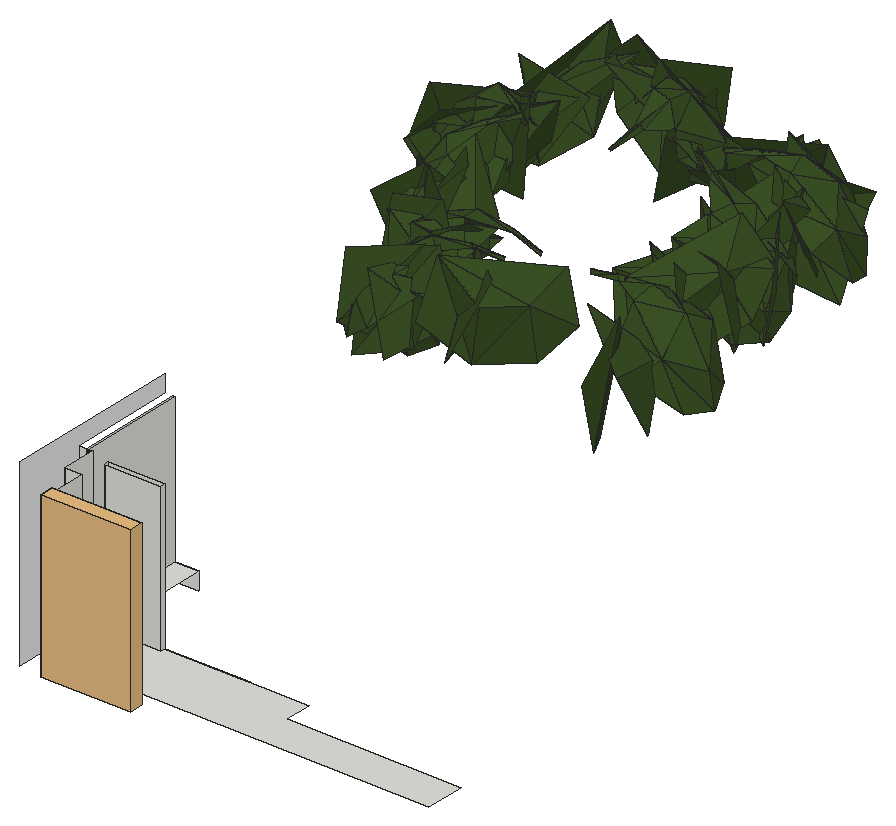
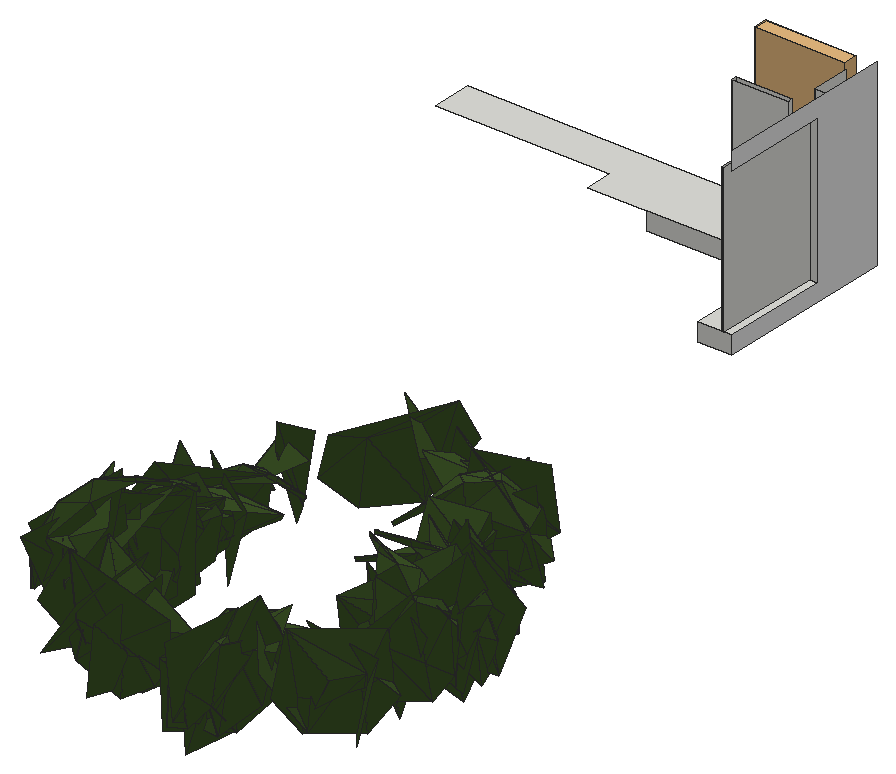
# SketchUp Ruby script. Lengths in inches.
U = 1.inch
M = Sketchup.active_model
def pt(a) = Geom::Point3d.new(a.map { |v| v * U })
def face(e, loops, mat)
  f = e.add_face(loops[0].map { |a| pt(a) })
  loops[1..].each { |l| e.add_face(l.map { |a| pt(a) }).erase! }
  f.material = f.back_material = mat if mat
  f
end
# faces: each face lists its corners as indices into pts; further lists are holes
def faces(e, pts, list, mat = nil) = list.each { |f| face(e, (f[0].is_a?(Array) ? f : [f]).map { |l| l.map { |i| pts[i] } }, mat) }
# xy, xz, yz: faces in a plane at the given z, y or x. An outline is a flat list of corners, or four numbers for a rectangle; further outlines are holes
def ring(l) = l.size == 4 ? [[l[0], l[1]], [l[2], l[1]], [l[2], l[3]], [l[0], l[3]]] : l.each_slice(2).to_a
def flat(e, list, mat, &to3) = list.each { |f| face(e, (f[0].is_a?(Array) ? f : [f]).map { |l| ring(l).map { |u, v| to3.(u, v) } }, mat) }
def xy(e, z, list, mat = nil) = flat(e, list, mat) { |x, y| [x, y, z] }
def xz(e, y, list, mat = nil) = flat(e, list, mat) { |x, z| [x, y, z] }
def yz(e, x, list, mat = nil) = flat(e, list, mat) { |y, z| [x, y, z] }
def lines(e, pts, list) = list.each { |a, b| e.add_line(pt(pts[a]), pt(pts[b])) }
# prism: a flat outline (further loops are holes) pulled along v
def prism(e, loops, v, mat = nil)
  f = face(e, loops, mat); d = Geom::Vector3d.new(v.map { |x| x * U })
  f.pushpull(f.normal.samedirection?(d) ? d.length : -d.length)
end
def box(e, o, s, mat = nil) = prism(e, [[o, [o[0] + s[0], o[1], o[2]], [o[0] + s[0], o[1] + s[1], o[2]], [o[0], o[1] + s[1], o[2]]]], [0, 0, s[2]], mat)
def at(x, y, z, deg = 0) = Geom::Transformation.translation(pt([x, y, z])) * Geom::Transformation.rotation(ORIGIN, Z_AXIS, deg.degrees)
def axes(o, x, y, z) = Geom::Transformation.new([*x, 0, *y, 0, *z, 0, *pt(o).to_a, 1])
def part(name) = M.definitions.add(name)
# library, detail: a bought-in or finely detailed component or shape, given as its bounding box
def library(name, o, s) = part(name).tap { |d| box(d.entities, o, s) }
def detail(e, o, s) = box(e.add_group.entities, o, s)
def put(e, d, t, mat = nil) = e.add_instance(d, t).tap { |i| i.material = mat if mat }
def group(e, t, mat = nil) = e.add_group.tap { |g| g.transformation = t; g.material = mat if mat }.entities
root = M.entities
M.materials.add("AM113_062_Tilia").color = [58, 81, 37]
M.materials.add("white_wall").color = [233, 233, 233]
c1 = library("Shrub+_Grass",[-121.83,-22.34,0],[123.96,19.94,123.95])
xy(root,297.35,[[413.32,28.625,935.92,28.625,935.92,83.29,695.48,83.29,695.48,121.6875,496.21,121.6875,496.21,115.3125,418.81,115.3125,418.81,278.26,385.62,278.26,385.62,130.3125,390.32,130.3125,390.32,82.67,413.32,82.67],[418.81,115.3125,496.21,121.6875],[371.87,130.3125,382.06,278.26],[382.06,130.3125,385.62,278.26]])
xz(root,82.67,[[390.32,297.35,413.32,500.91]])
xz(root,115.3125,[[418.81,297.35,496.21,500.91]])
xz(root,121.6875,[[496.21,273.04,613.65,297.35],[418.81,297.35,496.21,500.91]])
xz(root,130.3125,[[371.87,297.35,382.06,500.91],[382.06,297.35,385.62,500.91],[385.62,297.35,390.32,500.91]])
xz(root,278.26,[[371.87,273.04,418.81,297.35],[382.06,297.35,385.62,500.91]])
yz(root,371.87,[[28.625,273.04,28.625,525.1,278.26,525.1,278.26,500.91,130.3125,500.91,130.3125,297.35,278.26,297.35,278.26,273.04]],"white_wall")
yz(root,382.06,[[130.3125,297.35,278.26,500.91]])
yz(root,385.62,[[130.3125,297.35,278.26,500.91]])
yz(root,390.32,[[82.67,297.35,130.3125,500.91]])
yz(root,413.32,[[28.625,297.35,82.67,500.91]])
yz(root,418.81,[[115.3125,297.35,121.6875,500.91]])
yz(root,496.21,[[115.3125,297.35,121.6875,500.91]])
p = [[565.42,1074.05,347.14],[473.11,1076.04,429.39],[517.03,1076.78,251.14],[451.75,1104.5,310.63],[124.09,980.42,346.32],[174.26,1054.83,429.43],
  [142.82,1026.51,253.56],[201.08,1066.89,309.96],[542.4,803.89,256.72],[526.35,835.0625,255.56],[521.17,877.52,364.75],[204.78,925.17,256.16],
  [226.65,870.02,314.07],[218.93,918.58,365.5],[200.1875,963.85,327.84],[236.73,1028.86,315.61],[184.69,1005.02,258.76],[529.41,865.28,392.49],
  [539.14,787.86,344.57],[560.75,821.36,346.28],[565.625,868.44,257.36],[543.39,920.94,325.3],[557.08,902.7,333.4375],[580.49,912.46,269.3],
  [588.52,955.39,257.48],[585.34,950.82,307.52],[576.85,986.33,274.56],[268.35,895.48,383.67],[270.83,858.14,265.86],[220.66,790.14,270.84],
  [182.18,990.33,313.11],[157.6,954.42,268.03],[158.1,911.76,284.91],[196.71,1003.23,274.22],[140.53,985.93,269.15],[162.25,965.33,292.7],
  [127.97,985.77,316.2],[115.83,1037.13,348.44],[119.67,1023.7,279.89],[535.94,880.77,309],[440.12,1029.02,382.82],[481.72,1009.85,270.04],
  [536.36,947.3,290.85],[518.68,1039.48,342.86],[530.18,1055.24,275.41],[554.09,1092.74,270.55],[559.36,1077.5625,316.66],[561.57,1119.85,298.74],
  [232.85,789.04,384.3125],[140.57,950.14,352.37],[190.2,974.27,273.55],[236.15,982.17,351.65],[310.18,1219.3,383.75],[269.26,1249.37,274.58],
  [281.45,1333.08,273.91],[291.21,1329.84,387.71],[246.46,993.13,313.43],[555.97,993,341.74],[518.39,1024.73,340.52],[289.46,790.39,377.59],
  [237.56,799.57,345.67],[272.73,819.99,274.86],[332.7,798.7,318.77],[196.34,847.78,367.41],[191.52,826.9,289],[546.44,1120.36,421.7],
  [586.46,1062.82,356.48],[559.14,1076.29,275.13],[526.65,1124.94,400.61],[528.91,1091.98,285.93],[485.8,1034.11,325.7],[177.74,971.25,413.4],
  [105.18,966.85,356.36],[124.28,988.9,275.76],[189.57,987.47,392.76],[152.64,1007.23,285.1],[418.84,1319.11,379.39],[439.56,1305.13,276.45],
  [389.36,1247.37,293.16],[470.83,1253.625,285.62],[399.27,1259.62,276.43],[408.0625,1287.39,349.05],[354.28,1271.51,311.54],[480.33,1272.95,294.44],
  [408.32,1286.3,277.53],[409.71,1275.94,358.07],[361.54,1288.3,309.81],[516.07,1024.48,357.375],[499.64,1036.16,278.41],[486.36,1116.42,293.93],
  [147.64,925.03,291.07],[181.33,926.36,278.61],[241.63,929.63,372.95],[346.58,1295.18,353.86],[326.71,1314.76,278.91],[251.58,1282.1875,288.58],
  [255.6,805.6,278.97],[316.54,775.61,318.15],[288.3,803.46,381.79],[239.32,826.95,359.37],[222.83,900.29,359.07],[190.1875,851.45,304.82],
  [175.07,1024.77,279.71],[215.3,966.87,305.31],[177.61,975.15,368.4375],[142.8,1017.9,354.66],[140.06,1082.25,401.69],[116.41,1073.2,315.95],
  [125.43,1069.0625,333.45],[465.625,1034.93,394.92],[486.8,1025.62,306.64],[502.52,1104.04,281.29],[522.74,1072.12,354.01],[543.91,1122.28,375.93],
  [534.38,1165.23,317.22],[584.42,1102.64,358.01],[540.49,1142.12,281.66],[509.74,1172.49,364.83],[470.93,947.34,384.19],[493.29,929.2,309.82],
  [518.91,1004.47,282.71],[528,974.23,360.85],[547.36,1025.99,384.49],[551.39,1062.78,318.11],[176.99,893.1875,315.62],[163.21,934.92,325.15],
  [465.66,1291.55,358.61],[499.27,1261.56,420.2],[532.42,1274.12,350.76],[105.04,1045.5,364.82],[117.67,1058.8,286.46],[194.12,1032.34,290.86],
  [173.24,914.7,379.5],[197.41,877.89,287.8],[265.34,886.15,335.07],[198.48,1273.14,350.54],[242.27,1301.75,396.73],[285.03,1317.81,350.16],
  [204.99,1115.18,442.68],[201.84,1106.86,317.86],[133.52,1149.07,289.38],[103.75,1139,394.64],[346.81,1236.28,346.6],[342.13,1293.99,290.875],
  [260.27,1303.03,289.6],[298.73,1293.05,360.57],[201.45,1301.11,348.3125],[250.09,1290.84,398.875],[535.63,971.84,400.95],[177.58,965.8,356.21],
  [140.22,1001.44,324.09],[233.68,980.02,326.08],[232.74,931.4,404.49],[150.63,947.48,376.5625],[426.15,983.3,365.78],[468.47,935.03,323.04],
  [528.875,985.3,291.24],[501.21,983.41,371.14],[534.21,1028.18,387.43],[570.23,1042.13,322.73],[210.93,958.6,382.64],[164.91,963.76,364.36],
  [419.77,1201.3125,388.88],[442.71,1195.97,406.0625],[483.45,1217.41,293.45],[509.33,1297.54,303.9375],[539.3,1080.3125,324.46],[552.52,1127.77,364.5],
  [513.36,1173.52,338.95],[463.64,1266.77,378.92],[491.1875,1203.03,416.06],[531.48,1253.21,373.72],[523.09,1139.91,457.67],[519.49,1132.15,330.84],
  [591.36,1168.09,296.72],[595.41,1211.44,396.58],[148.9,1201.36,298.59],[130.5,1157.85,332.11],[127.95,1211.69,374.61],[169.52,1269.79,311.48],
  [259.3,769.38,400.81],[285.56,763.64,298.66],[338.32,812.03,337.35],[560.28,1116.76,371.51],[542.35,1158.59,395.58],[329.71,1300.86,345.54],
  [336.4,1283.18,306.22],[304.24,1336.92,301.48],[264.22,1351.13,319.19],[124.7,1215.33,303.35],[115.4375,1168.3,332.79],[140.02,1210.64,382.35],
  [153.0625,1282.39,323.1],[580.81,1243.58,398.83],[545.72,1225.25,303.81],[484.52,1220.6,365.09],[451.14,1307.125,389.6],[219.18,765.42,320.9],
  [241.2,789.54,304.42],[299.26,826.3,388.73],[206.67,835.57,354.34],[203.98,795.28,304.625],[234.38,762.87,310.03],[202.77,857.17,317.74],
  [222.12,933.99,356.98],[148.71,1116.59,306.13],[116.23,1054.54,333.8],[122.6,1086.16,402.59],[145.76,1136.13,388.46],[211.85,1159.8125,418.71],
  [178.29,1185.79,345.08],[309.91,1239.64,345],[100.96,1226.86,409.14],[112.4375,1249.61,306.4],[159.93,1188.44,313.2],[547.72,956.81,363.52],
  [83.67,1111.39,403.31],[107.58,1083.3,308.36],[146.61,1037.31,368.88],[335.17,861.17,413.37],[346.14,806.08,308.68],[389.2,738.24,342.82],
  [494.05,913.92,341.8125],[164.55,1101.23,309.81],[138.74,1041.11,345.54],[111.78,1083.61,393.14],[124.02,1134.8,363.83],[158.99,1180.49,401.77],
  [159.98,1181.6875,319.94],[353.26,1227.36,351.68],[265.27,759.75,332.54],[230.01,781.04,354.46],[560.0625,995,414.84],[575.67,1007.41,310.08],
  [538.94,1073.21,334.06],[382.68,793.49,313.49],[432.64,845.53,311.05],[435.63,828.28,389.64],[463.07,876.98,351.67],[135.91,1268.4,388.18],
  [358.56,1263.54,380.97],[175.64,1292.39,448.04],[165.7,1330.77,382.49],[559.6,1109.25,440.05],[600.6,1117.37,364.04],[554.76,1172.62,311.98],
  [572.07,1175.27,396.56],[515.52,1234.72,327.23],[539.12,1221.7,401.12],[280.37,1356.24,325.22],[269.76,1324.34,312.32],[252.59,1265.63,405.83],
  [204.46,956.31,369.4],[247.74,991.84,351.14],[216.8,1204.48,404.96],[347.79,778.22,444.4375],[349.14,738.3125,379.18],[401.84,781.17,396.57],
  [237.98,860.38,379.8125],[99.35,1133.52,314.8],[93.3,1103.35,336.5],[103.99,1140.44,363.4],[152.11,1168.9,385.16],[127.88,1166.51,321.61],
  [597.96,1153.28,398.18],[609.04,1168.27,330.3125],[594.16,1208.65,315.06],[597.12,1206.875,365.41],[570.08,1231.25,332.27],[202.74,915.69,373.65],
  [245.96,893.42,383.27],[286.1,906.75,404.6],[145.5,995.08,384.94],[541.24,1082.78,387.08],[559.46,1182.5,373.32],[252.48,880.33,346.4],
  [341.91,771.98,378.12],[564.95,1086.46,378.09],[352.45,786.75,381.62],[284.49,1337.82,358.91],[240.5,1339.56,350.03],[296.76,819.8,421.14],
  [221.16,778.91,409.52],[181.27,1174.29,360.42],[577.08,1072.7,378.02],[160.95,1260.6,405.38],[230.96,1273.36,436.63],[187.35,1324.65,402.84],
  [257.62,1273,437.4375],[301.08,1344.65,410.22],[466.5,888.41,376.58],[471.67,1070.36,383.2],[233.24,941.21,372.79],[501.54,1267.84,377.62],
  [588.67,1122.17,378.51],[143.38,1157.01,400.51],[553.38,1232.02,401.89],[505.17,1241.48,405.11],[279.51,790.07,391.25],[327.29,801.63,388.86],
  [175.88,1146.29,366.84],[497.9,928.74,374.03],[167.03,1061.3,385.09],[99.37,1030.38,389.49],[458.14,1049.2,383.12],[273.53,975.64,363.21],
  [122.52,1047.93,411.18],[107.01,1093.55,404.89],[291.87,882.28,386.62],[547.34,1187.59,389.81],[493.73,986.29,341.62],[507.53,977.93,373.27],
  [417.13,785.98,432.45],[488.14,1073.95,414.11],[325.2,984.35,344.57],[283.95,985.58,358.36],[288.24,983.82,365.24],[326.75,985.04,349.57],
  [308.58,1238.47,382.72],[112.97,1021.65,399.88],[290.53,1291.21,402.21],[260.47,877.93,382.625],[291.24,978.7,363.01],[325.64,981.89,346.5],
  [215.91,1231.58,437.36],[189.03,1293.11,414.09],[164.44,1043.63,414.3],[217.24,1274.08,416.8],[253.1,1306.93,407.28],[187.52,1275.17,418.59],
  [245.63,975.03,378.875],[442.29,884.58,416.02],[192.7,1035.61,428.46],[231.34,1267.91,459.49],[254.15,821.66,397.31],[261.98,930.65,356.1],
  [248.65,947.68,381.73],[198.66,949.72,424.68],[234.41,972.27,428.45],[555.38,1148.27,437.51],[481.42,1101.7,432.33],[351.98,836.91,407.47],
  [199.45,1128.51,400.53],[132.23,1121.73,422.3125],[321.45,924.22,363.5],[292.43,896.89,382.99],[297.86,898.01,388.64],[322.98,925.46,368.32],
  [506.06,952.68,387.53],[207.64,1002.96,391.28],[184.85,998.7,413.5625],[302.99,896.34,384.74],[323.67,922.57,364.68],[506.97,1161.17,451.78],
  [565.46,1198.15,426.71],[515.01,1099.81,398.31],[325.29,810.4375,434.49],[194.16,1090.85,441.4],[310.88,841.6,369.74],[294.375,843.85,400.94],
  [422.66,949.15,371.29],[464.48,944.32,380],[461.45,949.2,385.33],[421.69,950.66,376.23],[458.99,953.45,380.49],[422.84,952.05,371.48],
  [518.48,1113.59,420],[504.13,1133.78,399.64],[517.92,1169.01,443.11],[287.0625,1203.15,396.46],[274.65,1166.81,380.29],[274.5,1168.56,375.32],
  [290.15,1206.64,389.6],[281.2,1202.15,394.3],[272.05,1168.98,377.29],[471.86,1229.28,441.6875],[533.66,1071.42,432.41],[538.39,1133.32,416.1],
  [274.21,862.35,405.61],[293.79,1246,410.8],[168.35,1018.33,425.16],[188.42,1121.08,433.54],[508.65,1088.55,427.96],[246.32,1246.4,388.7],
  [267.14,1252.67,414.16],[152.27,1027.71,445.43],[118.4375,1051.59,457],[536.71,1150.49,446.64],[502.68,1196.2,412.1875],[520.94,1197.92,441.77],
  [162.87,1067.77,409.6],[155.26,1084.7,438.2],[205.64,1044.02,439.63],[467.88,1098.36,439.08],[196.58,1048.49,435.96],[467.4375,1108.24,444.23],
  [169.26,1106.42,449.04],[200.24,1045.59,442.625],[533.01,1176.29,457.45],[468.58,1102.42,446.49],[208.61,1091.75,444.42],[232.63,1068.24,446.92],
  [208.57,1081.38,446.56],[432.64,1120.08,452.24],[232.97,1066.99,452.02],[234.07,1065.77,447.26],[208.63,1086.64,450.52],[241.46,1064.52,445.45],
  [241.45,1065.8,440.34],[239.8125,1063.48,440.875],[491.32,1153.76,458.05],[433.5,1120.53,457.55],[434.15,1122.5,452.98],[500.52,1148.41,457.15],
  [495.88,1151.6,462.67],[460.05,1133.04,460.01],[461.28,1131.82,455.03],[460.03,1134.46,455.04]]
faces(root,p,[[0,1,2],[1,3,2],[4,5,6],[5,7,6],[8,9,10],[11,12,13],[13,14,11],[15,16,11],
  [11,14,15],[17,18,8],[10,17,8],[19,20,21],[22,23,24],[24,25,22],[24,26,25],[27,28,29],
  [30,31,32],[30,33,31],[34,35,36],[34,36,37],[37,38,34],[22,39,23],[40,41,42],[43,44,45],
  [45,46,43],[45,47,46],[48,27,29],[49,50,51],[52,53,54],[55,52,54],[56,33,30],[25,26,57],
  [26,58,57],[59,60,61],[61,62,59],[61,60,63],[63,64,61],[65,66,67],[68,65,67],[67,69,68],
  [43,70,44],[71,72,73],[74,71,73],[73,75,74],[76,77,78],[79,80,81],[80,82,81],[83,84,85],
  [84,86,85],[87,88,89],[90,91,92],[93,94,95],[96,97,98],[98,99,96],[100,101,96],[96,99,100],
  [102,103,104],[104,105,102],[102,105,106],[106,107,102],[37,108,38],[109,110,111],[111,112,109],[113,112,111],
  [111,114,113],[115,116,117],[118,119,120],[120,121,118],[122,121,120],[120,123,122],[32,124,125],[32,125,30],
  [81,126,79],[79,126,127],[127,128,79],[129,130,131],[132,133,134],[95,135,136],[136,137,95],[95,137,93],
  [138,139,140],[141,138,140],[142,143,144],[144,145,142],[144,146,147],[147,145,144],[148,40,42],[149,150,131],
  [131,151,149],[131,150,129],[92,152,90],[152,153,90],[154,155,156],[156,157,154],[158,157,156],[156,159,158],
  [35,160,161],[36,35,161],[76,78,162],[163,164,165],[89,166,87],[167,166,89],[89,168,167],[83,169,170],
  [170,171,83],[85,169,83],[172,173,174],[175,172,174],[176,177,178],[179,176,178],[180,181,182],[46,47,183],
  [47,184,183],[185,186,187],[185,187,188],[189,190,191],[192,189,191],[193,194,195],[196,163,165],[197,198,199],
  [200,201,202],[200,203,201],[103,204,104],[205,206,207],[207,208,205],[205,208,209],[209,210,205],[211,186,185],
  [212,213,214],[22,25,215],[215,25,57],[216,217,218],[219,220,221],[222,39,22],[223,224,225],[225,226,223],
  [223,226,227],[227,228,223],[85,86,229],[202,230,231],[202,231,200],[232,233,234],[235,236,237],[236,238,237],
  [178,239,179],[81,82,240],[179,239,241],[241,242,179],[243,244,245],[245,246,243],[245,247,248],[248,246,245],
  [249,250,251],[30,125,252],[253,30,252],[30,253,56],[212,214,254],[255,256,235],[235,257,255],[237,257,235],
  [12,258,13],[259,260,261],[262,263,259],[259,261,262],[264,265,266],[266,267,264],[266,268,267],[125,124,269],
  [124,270,269],[13,271,15],[15,14,13],[272,36,161],[37,36,272],[43,46,273],[273,46,183],[114,274,113],
  [275,203,200],[97,276,98],[123,277,122],[62,278,59],[188,279,185],[188,280,279],[199,281,197],[281,282,197],
  [262,283,263],[159,284,158],[191,285,192],[192,285,286],[286,287,192],[129,150,149],[87,166,167],[252,125,269],
  [251,288,249],[288,289,249],[19,21,290],[291,70,43],[151,292,149],[247,293,248],[264,294,265],[178,177,295],
  [267,268,296],[268,297,296],[231,230,298],[230,299,298],[191,190,300],[22,301,222],[301,22,215],[302,108,37],
  [206,303,207],[232,234,304],[132,134,305],[260,306,307],[261,260,307],[180,182,308],[168,309,167],[57,58,310],
  [310,311,57],[215,57,311],[312,219,221],[43,313,291],[313,43,273],[314,315,316],[316,317,314],[185,318,211],
  [224,319,225],[318,185,320],[185,279,320],[63,60,59],[200,321,275],[322,323,317],[147,324,142],[142,145,147],
  [146,325,147],[326,37,272],[37,326,302],[81,240,127],[127,126,81],[317,316,322],[280,327,328],[279,280,328],
  [93,137,136],[135,329,136],[252,330,253],[315,253,330],[237,238,331],[49,51,332],[85,229,170],[136,333,93],
  [109,112,113],[200,231,334],[321,200,334],[334,231,298],[106,105,104],[269,270,335],[335,336,269],[149,292,337],
  [149,337,129],[104,204,338],[167,339,87],[115,117,340],[170,169,85],[330,316,315],[320,279,328],[98,341,100],
  [100,99,98],[342,283,262],[118,121,122],[330,336,322],[322,316,330],[343,261,307],[262,261,343],[344,345,346],
  [346,347,344],[215,348,301],[215,311,348],[227,226,225],[161,160,349],[272,161,350],[349,350,161],[167,309,339],
  [351,352,347],[193,195,353],[264,267,354],[354,267,296],[13,258,271],[158,355,154],[154,157,158],[191,300,286],
  [59,356,63],[347,346,351],[104,338,106],[216,218,357],[252,269,336],[252,336,330],[298,299,358],[358,359,298],
  [360,361,362],[362,363,360],[364,365,363],[273,183,366],[367,366,183],[183,184,367],[348,311,364],[113,274,368],
  [361,301,348],[178,295,241],[241,239,178],[369,370,371],[371,372,369],[113,368,109],[363,362,364],[373,374,370],
  [59,278,356],[248,293,375],[158,284,355],[98,276,341],[122,277,376],[377,294,264],[348,362,361],[370,369,373],
  [364,362,348],[286,285,191],[334,378,321],[345,321,378],[372,318,379],[320,379,318],[378,346,345],[122,376,118],
  [378,359,351],[351,346,378],[272,350,380],[272,380,326],[381,262,343],[262,381,342],[273,382,313],[273,366,382],
  [209,208,207],[328,327,383],[383,384,328],[207,303,385],[237,331,255],[255,257,237],[379,369,372],[334,298,359],
  [225,319,386],[225,386,227],[379,384,373],[373,369,379],[243,246,248],[136,329,333],[334,359,378],[264,387,377],
  [387,264,354],[147,325,324],[248,375,243],[296,297,388],[388,389,296],[354,296,389],[320,384,379],[320,328,384],
  [207,385,209],[307,306,390],[390,391,307],[343,307,391],[380,350,392],[393,313,382],[394,326,380],[382,366,395],
  [343,391,396],[343,396,381],[392,397,380],[380,397,394],[354,398,387],[354,389,398],[395,399,382],[382,399,393],
  [400,381,396],[401,394,397],[396,391,402],[403,393,399],[404,397,392],[392,405,404],[406,407,408],[408,400,406],
  [402,409,407],[398,389,410],[397,404,401],[411,399,395],[395,412,411],[396,406,400],[407,406,402],[399,411,403],
  [402,406,396],[413,387,398],[414,415,416],[416,413,414],[410,417,415],[398,414,413],[410,414,398],[415,414,410]],"AM113_062_Tilia")
put(root,c1,axes([537.6,31.03,284.22],[1,0,0],[0,1,0],[0,0,1.815]))
